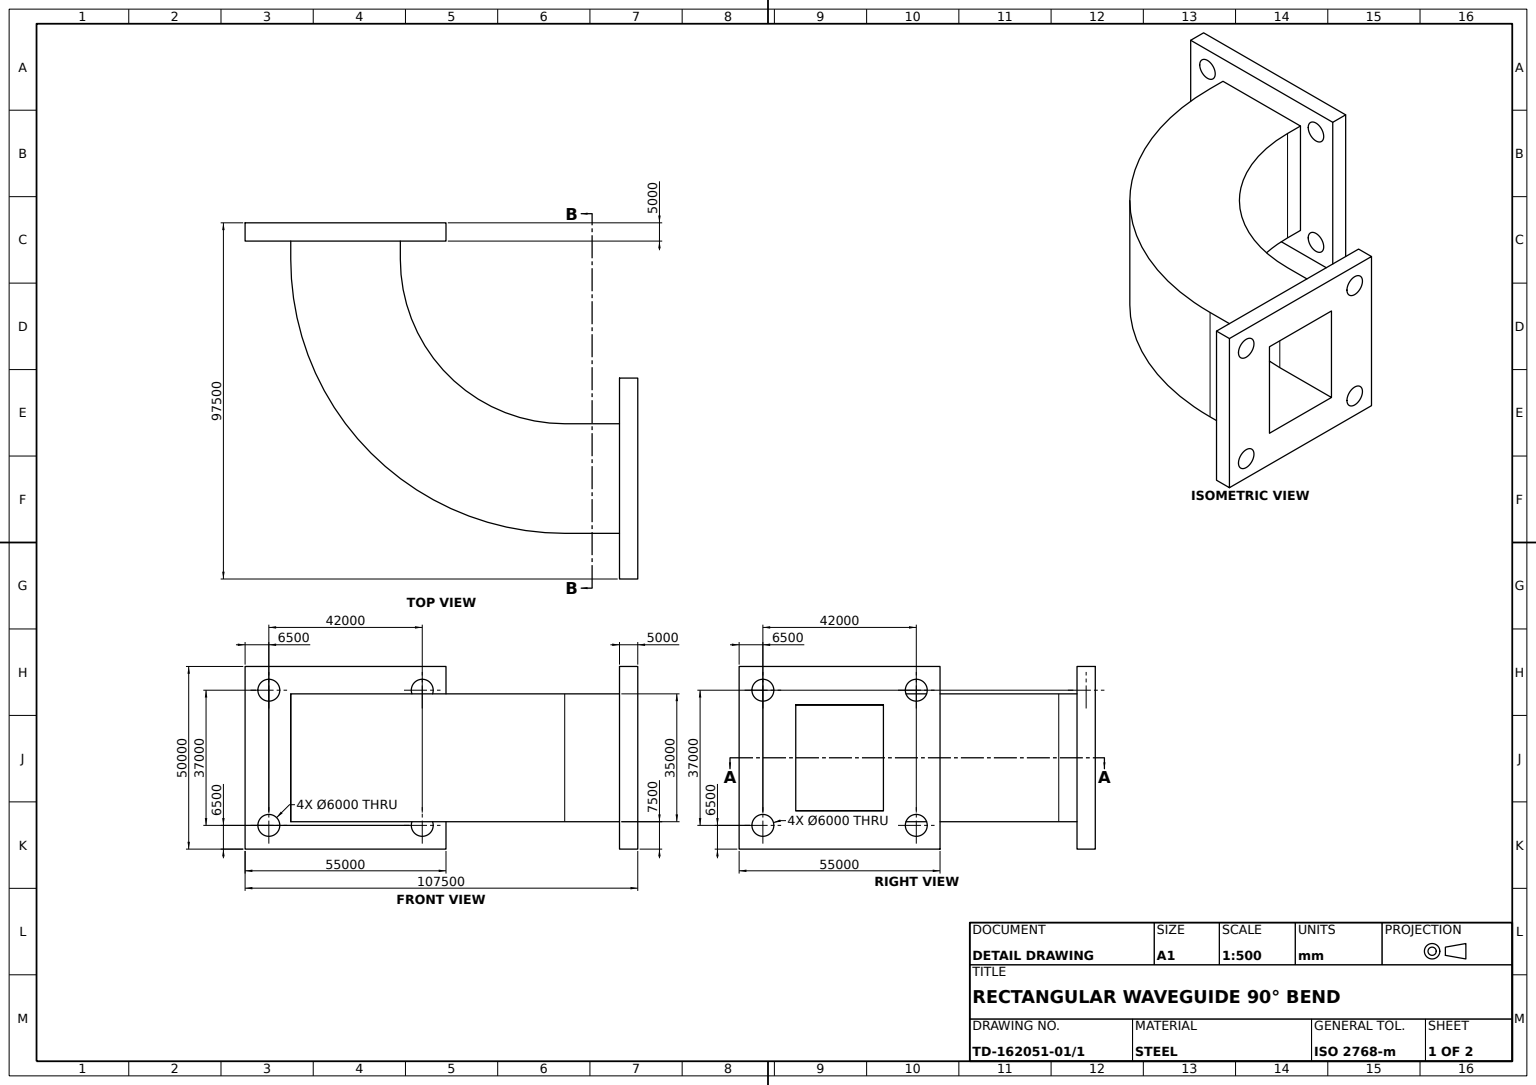
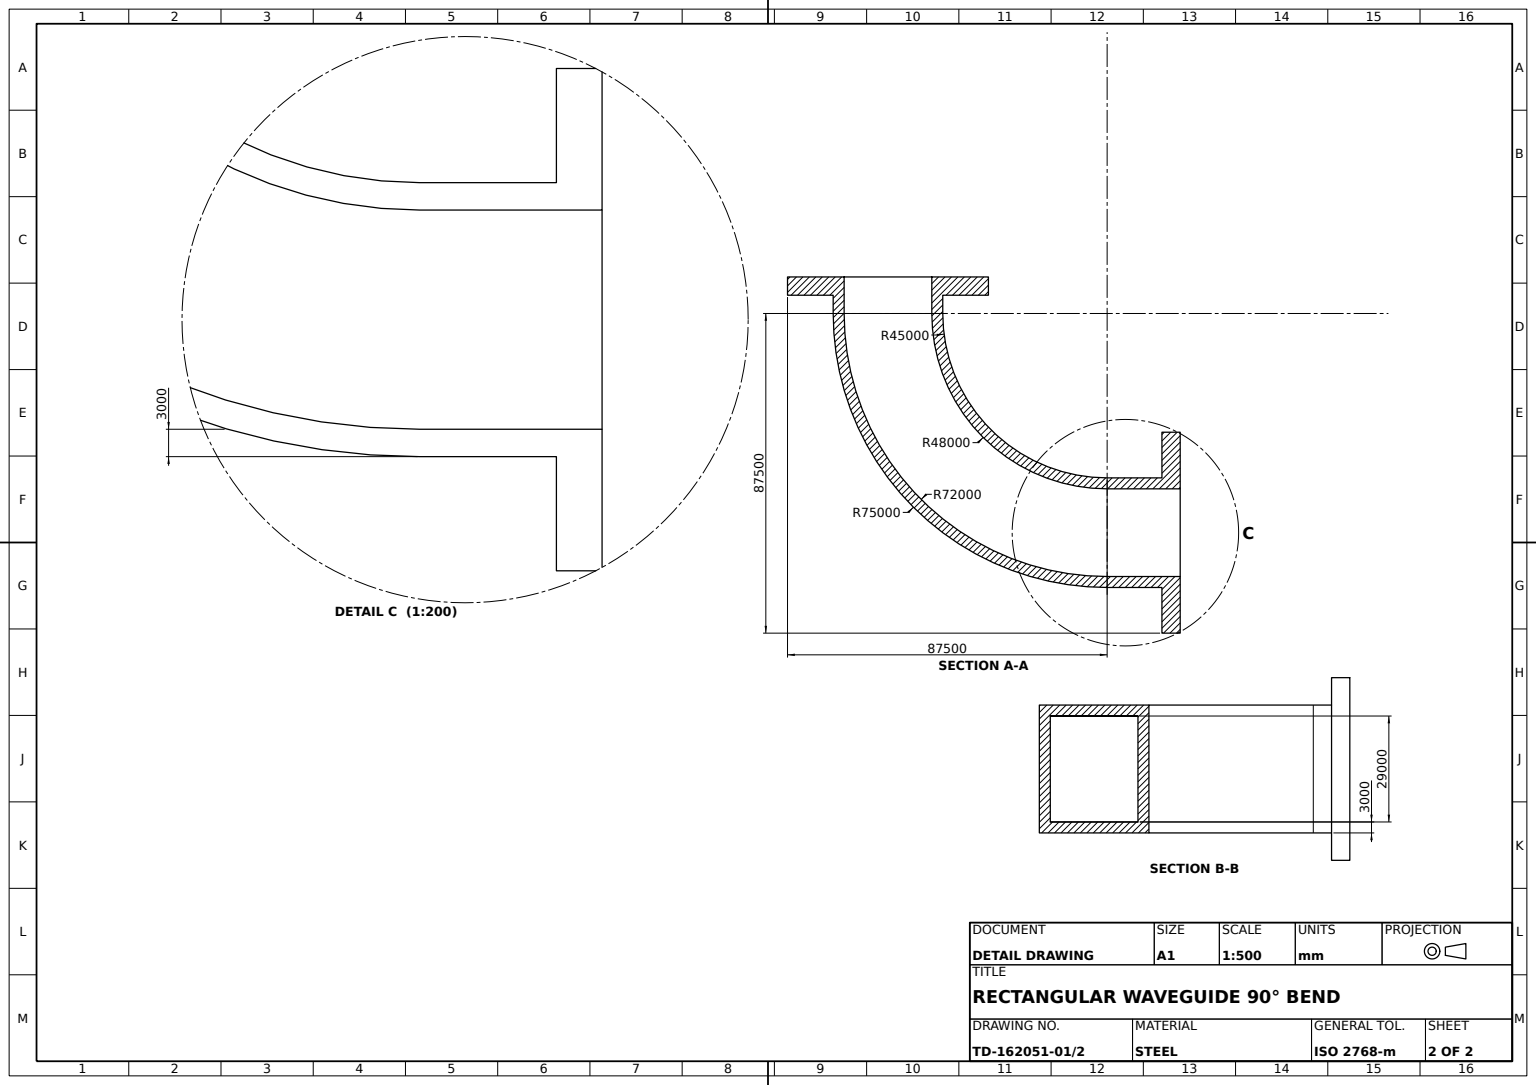
ISO-10303-21;
HEADER;
FILE_DESCRIPTION((''),'2;1');
FILE_NAME('','',(''),(''),'','','');
FILE_SCHEMA(('AUTOMOTIVE_DESIGN'));
ENDSEC;
DATA;
#1=APPLICATION_CONTEXT('');
#2=PRODUCT_CONTEXT('',#1,'mechanical');
#3=PRODUCT('','','',(#2));
#4=PRODUCT_DEFINITION_FORMATION('','',#3);
#5=PRODUCT_DEFINITION_CONTEXT('',#1,'design');
#6=PRODUCT_DEFINITION('','',#4,#5);
#7=PRODUCT_DEFINITION_SHAPE('','',#6);
#8=(LENGTH_UNIT()NAMED_UNIT(*)SI_UNIT(.MILLI.,.METRE.));
#9=(NAMED_UNIT(*)PLANE_ANGLE_UNIT()SI_UNIT($,.RADIAN.));
#10=(NAMED_UNIT(*)SI_UNIT($,.STERADIAN.)SOLID_ANGLE_UNIT());
#11=UNCERTAINTY_MEASURE_WITH_UNIT(LENGTH_MEASURE(1.E-05),#8,'distance_accuracy_value','');
#12=(GEOMETRIC_REPRESENTATION_CONTEXT(3)GLOBAL_UNCERTAINTY_ASSIGNED_CONTEXT((#11))GLOBAL_UNIT_ASSIGNED_CONTEXT((#8,#9,#10))REPRESENTATION_CONTEXT('',''));
#13=CARTESIAN_POINT('',(89000.,-18500.,-80000.));
#14=VERTEX_POINT('',#13);
#15=CARTESIAN_POINT('',(83000.,-18500.,-80000.));
#16=VERTEX_POINT('',#15);
#17=CARTESIAN_POINT('',(86000.,-18500.,-80000.));
#18=DIRECTION('',(0.,0.,-1.));
#19=DIRECTION('',(-1.,0.,0.));
#20=AXIS2_PLACEMENT_3D('',#17,#18,#19);
#21=CIRCLE('',#20,3000.);
#22=EDGE_CURVE('',#14,#16,#21,.T.);
#23=ORIENTED_EDGE('',*,*,#22,.T.);
#24=CARTESIAN_POINT('',(83000.,-18500.,-75000.));
#25=VERTEX_POINT('',#24);
#26=CARTESIAN_POINT('',(83000.,-18500.,27500.001));
#27=VECTOR('',#18,1000.);
#28=LINE('',#26,#27);
#29=EDGE_CURVE('',#25,#16,#28,.T.);
#30=ORIENTED_EDGE('',*,*,#29,.F.);
#31=CARTESIAN_POINT('',(89000.,-18500.,-75000.));
#32=VERTEX_POINT('',#31);
#33=CARTESIAN_POINT('',(86000.,-18500.,-75000.));
#34=DIRECTION('',(0.,0.,1.));
#35=AXIS2_PLACEMENT_3D('',#33,#34,#19);
#36=CIRCLE('',#35,3000.);
#37=EDGE_CURVE('',#25,#32,#36,.T.);
#38=ORIENTED_EDGE('',*,*,#37,.T.);
#39=CARTESIAN_POINT('',(89000.,-18500.,27500.001));
#40=LINE('',#39,#27);
#41=EDGE_CURVE('',#32,#14,#40,.T.);
#42=ORIENTED_EDGE('',*,*,#41,.T.);
#43=EDGE_LOOP('',(#23,#30,#38,#42));
#44=FACE_OUTER_BOUND('',#43,.T.);
#45=CARTESIAN_POINT('',(86000.,-18500.,27500.001));
#46=AXIS2_PLACEMENT_3D('',#45,#18,#19);
#47=CYLINDRICAL_SURFACE('',#46,3000.);
#48=ADVANCED_FACE('',(#44),#47,.F.);
#49=CARTESIAN_POINT('',(50000.,-17500.,-60000.));
#50=VERTEX_POINT('',#49);
#51=CARTESIAN_POINT('',(50000.,-17500.,-75000.));
#52=VERTEX_POINT('',#51);
#53=LINE('',#49,#27);
#54=EDGE_CURVE('',#50,#52,#53,.T.);
#55=ORIENTED_EDGE('',*,*,#54,.F.);
#56=CARTESIAN_POINT('',(50000.,17500.,-60000.));
#57=VERTEX_POINT('',#56);
#58=CARTESIAN_POINT('',(50000.,14500.,-60000.));
#59=DIRECTION('',(0.,1.,0.));
#60=VECTOR('',#59,1000.);
#61=LINE('',#58,#60);
#62=EDGE_CURVE('',#50,#57,#61,.T.);
#63=ORIENTED_EDGE('',*,*,#62,.T.);
#64=CARTESIAN_POINT('',(50000.,17500.,-75000.));
#65=VERTEX_POINT('',#64);
#66=LINE('',#56,#27);
#67=EDGE_CURVE('',#57,#65,#66,.T.);
#68=ORIENTED_EDGE('',*,*,#67,.T.);
#69=CARTESIAN_POINT('',(50000.,0.,-75000.));
#70=LINE('',#69,#60);
#71=EDGE_CURVE('',#52,#65,#70,.T.);
#72=ORIENTED_EDGE('',*,*,#71,.F.);
#73=EDGE_LOOP('',(#55,#63,#68,#72));
#74=FACE_OUTER_BOUND('',#73,.T.);
#75=DIRECTION('',(0.,-1.,0.));
#76=AXIS2_PLACEMENT_3D('',#58,#19,#75);
#77=PLANE('',#76);
#78=ADVANCED_FACE('',(#74),#77,.T.);
#79=CARTESIAN_POINT('',(80000.,-17500.,-60000.));
#80=VERTEX_POINT('',#79);
#81=CARTESIAN_POINT('',(77000.,-17500.,-60000.));
#82=VECTOR('',#19,1000.);
#83=LINE('',#81,#82);
#84=EDGE_CURVE('',#80,#50,#83,.T.);
#85=ORIENTED_EDGE('',*,*,#84,.F.);
#86=CARTESIAN_POINT('',(5000.,-17500.,15000.));
#87=VERTEX_POINT('',#86);
#88=CARTESIAN_POINT('',(5000.,-17500.,-60000.));
#89=AXIS2_PLACEMENT_3D('',#88,#59,#18);
#90=CIRCLE('',#89,75000.);
#91=EDGE_CURVE('',#87,#80,#90,.T.);
#92=ORIENTED_EDGE('',*,*,#91,.F.);
#93=CARTESIAN_POINT('',(5000.,-17500.,-15000.));
#94=VERTEX_POINT('',#93);
#95=CARTESIAN_POINT('',(5000.,-17500.,12000.));
#96=LINE('',#95,#27);
#97=EDGE_CURVE('',#87,#94,#96,.T.);
#98=ORIENTED_EDGE('',*,*,#97,.T.);
#99=CIRCLE('',#89,45000.);
#100=EDGE_CURVE('',#94,#50,#99,.T.);
#101=ORIENTED_EDGE('',*,*,#100,.T.);
#102=EDGE_LOOP('',(#85,#92,#98,#101));
#103=FACE_OUTER_BOUND('',#102,.T.);
#104=AXIS2_PLACEMENT_3D('',#95,#75,#18);
#105=PLANE('',#104);
#106=ADVANCED_FACE('',(#103),#105,.T.);
#107=CARTESIAN_POINT('',(0.,-18500.,-24000.));
#108=VERTEX_POINT('',#107);
#109=CARTESIAN_POINT('',(0.,-18500.,-18000.));
#110=VERTEX_POINT('',#109);
#111=CARTESIAN_POINT('',(0.,-18500.,-21000.));
#112=DIRECTION('',(1.,0.,0.));
#113=AXIS2_PLACEMENT_3D('',#111,#112,#34);
#114=CIRCLE('',#113,3000.);
#115=EDGE_CURVE('',#108,#110,#114,.T.);
#116=ORIENTED_EDGE('',*,*,#115,.T.);
#117=CARTESIAN_POINT('',(-5000.,-18500.,-18000.));
#118=VERTEX_POINT('',#117);
#119=CARTESIAN_POINT('',(92500.001,-18500.,-18000.));
#120=LINE('',#119,#82);
#121=EDGE_CURVE('',#110,#118,#120,.T.);
#122=ORIENTED_EDGE('',*,*,#121,.T.);
#123=CARTESIAN_POINT('',(-5000.,-18500.,-24000.));
#124=VERTEX_POINT('',#123);
#125=CARTESIAN_POINT('',(-5000.,-18500.,-21000.));
#126=AXIS2_PLACEMENT_3D('',#125,#19,#34);
#127=CIRCLE('',#126,3000.);
#128=EDGE_CURVE('',#118,#124,#127,.T.);
#129=ORIENTED_EDGE('',*,*,#128,.T.);
#130=CARTESIAN_POINT('',(92500.001,-18500.,-24000.));
#131=LINE('',#130,#82);
#132=EDGE_CURVE('',#108,#124,#131,.T.);
#133=ORIENTED_EDGE('',*,*,#132,.F.);
#134=EDGE_LOOP('',(#116,#122,#129,#133));
#135=FACE_OUTER_BOUND('',#134,.T.);
#136=CARTESIAN_POINT('',(92500.001,-18500.,-21000.));
#137=AXIS2_PLACEMENT_3D('',#136,#19,#34);
#138=CYLINDRICAL_SURFACE('',#137,3000.);
#139=ADVANCED_FACE('',(#135),#138,.F.);
#140=CARTESIAN_POINT('',(0.,17500.,15000.));
#141=VERTEX_POINT('',#140);
#142=CARTESIAN_POINT('',(0.,-17500.,15000.));
#143=VERTEX_POINT('',#142);
#144=CARTESIAN_POINT('',(0.,0.,15000.));
#145=VECTOR('',#75,1000.);
#146=LINE('',#144,#145);
#147=EDGE_CURVE('',#141,#143,#146,.T.);
#148=ORIENTED_EDGE('',*,*,#147,.F.);
#149=CARTESIAN_POINT('',(0.,17500.,-15000.));
#150=VERTEX_POINT('',#149);
#151=CARTESIAN_POINT('',(0.,17500.,0.));
#152=VECTOR('',#34,1000.);
#153=LINE('',#151,#152);
#154=EDGE_CURVE('',#150,#141,#153,.T.);
#155=ORIENTED_EDGE('',*,*,#154,.F.);
#156=CARTESIAN_POINT('',(0.,-17500.,-15000.));
#157=VERTEX_POINT('',#156);
#158=CARTESIAN_POINT('',(0.,0.,-15000.));
#159=LINE('',#158,#60);
#160=EDGE_CURVE('',#157,#150,#159,.T.);
#161=ORIENTED_EDGE('',*,*,#160,.F.);
#162=CARTESIAN_POINT('',(0.,-17500.,0.));
#163=LINE('',#162,#27);
#164=EDGE_CURVE('',#143,#157,#163,.T.);
#165=ORIENTED_EDGE('',*,*,#164,.F.);
#166=EDGE_LOOP('',(#148,#155,#161,#165));
#167=FACE_BOUND('',#166,.T.);
#168=CARTESIAN_POINT('',(0.,-25000.,-27500.));
#169=VERTEX_POINT('',#168);
#170=CARTESIAN_POINT('',(0.,-25000.,27500.));
#171=VERTEX_POINT('',#170);
#172=LINE('',#168,#152);
#173=EDGE_CURVE('',#169,#171,#172,.T.);
#174=ORIENTED_EDGE('',*,*,#173,.F.);
#175=CARTESIAN_POINT('',(0.,25000.,-27500.));
#176=VERTEX_POINT('',#175);
#177=LINE('',#175,#145);
#178=EDGE_CURVE('',#176,#169,#177,.T.);
#179=ORIENTED_EDGE('',*,*,#178,.F.);
#180=CARTESIAN_POINT('',(0.,25000.,27500.));
#181=VERTEX_POINT('',#180);
#182=LINE('',#175,#27);
#183=EDGE_CURVE('',#181,#176,#182,.T.);
#184=ORIENTED_EDGE('',*,*,#183,.F.);
#185=LINE('',#180,#60);
#186=EDGE_CURVE('',#171,#181,#185,.T.);
#187=ORIENTED_EDGE('',*,*,#186,.F.);
#188=EDGE_LOOP('',(#174,#179,#184,#187));
#189=FACE_OUTER_BOUND('',#188,.T.);
#190=ORIENTED_EDGE('',*,*,#115,.F.);
#191=EDGE_CURVE('',#110,#108,#114,.T.);
#192=ORIENTED_EDGE('',*,*,#191,.F.);
#193=EDGE_LOOP('',(#190,#192));
#194=FACE_BOUND('',#193,.T.);
#195=CARTESIAN_POINT('',(0.,18500.,18000.));
#196=VERTEX_POINT('',#195);
#197=CARTESIAN_POINT('',(0.,18500.,24000.));
#198=VERTEX_POINT('',#197);
#199=CARTESIAN_POINT('',(0.,18500.,21000.));
#200=AXIS2_PLACEMENT_3D('',#199,#112,#34);
#201=CIRCLE('',#200,3000.);
#202=EDGE_CURVE('',#196,#198,#201,.T.);
#203=ORIENTED_EDGE('',*,*,#202,.F.);
#204=EDGE_CURVE('',#198,#196,#201,.T.);
#205=ORIENTED_EDGE('',*,*,#204,.F.);
#206=EDGE_LOOP('',(#203,#205));
#207=FACE_BOUND('',#206,.T.);
#208=CARTESIAN_POINT('',(0.,18500.,-24000.));
#209=VERTEX_POINT('',#208);
#210=CARTESIAN_POINT('',(0.,18500.,-18000.));
#211=VERTEX_POINT('',#210);
#212=CARTESIAN_POINT('',(0.,18500.,-21000.));
#213=AXIS2_PLACEMENT_3D('',#212,#112,#34);
#214=CIRCLE('',#213,3000.);
#215=EDGE_CURVE('',#209,#211,#214,.T.);
#216=ORIENTED_EDGE('',*,*,#215,.F.);
#217=EDGE_CURVE('',#211,#209,#214,.T.);
#218=ORIENTED_EDGE('',*,*,#217,.F.);
#219=EDGE_LOOP('',(#216,#218));
#220=FACE_BOUND('',#219,.T.);
#221=CARTESIAN_POINT('',(0.,-18500.,24000.));
#222=VERTEX_POINT('',#221);
#223=CARTESIAN_POINT('',(0.,-18500.,18000.));
#224=VERTEX_POINT('',#223);
#225=CARTESIAN_POINT('',(0.,-18500.,21000.));
#226=AXIS2_PLACEMENT_3D('',#225,#112,#34);
#227=CIRCLE('',#226,3000.);
#228=EDGE_CURVE('',#222,#224,#227,.T.);
#229=ORIENTED_EDGE('',*,*,#228,.F.);
#230=EDGE_CURVE('',#224,#222,#227,.T.);
#231=ORIENTED_EDGE('',*,*,#230,.F.);
#232=EDGE_LOOP('',(#229,#231));
#233=FACE_BOUND('',#232,.T.);
#234=CARTESIAN_POINT('',(0.,0.,0.));
#235=AXIS2_PLACEMENT_3D('',#234,#19,#34);
#236=PLANE('',#235);
#237=ADVANCED_FACE('',(#167,#189,#194,#207,#220,#233),#236,.F.);
#238=CARTESIAN_POINT('',(80000.,17500.,-60000.));
#239=VERTEX_POINT('',#238);
#240=CARTESIAN_POINT('',(80000.,17500.,-75000.));
#241=VERTEX_POINT('',#240);
#242=LINE('',#238,#27);
#243=EDGE_CURVE('',#239,#241,#242,.T.);
#244=ORIENTED_EDGE('',*,*,#243,.F.);
#245=CARTESIAN_POINT('',(80000.,14500.,-60000.));
#246=LINE('',#245,#145);
#247=EDGE_CURVE('',#239,#80,#246,.T.);
#248=ORIENTED_EDGE('',*,*,#247,.T.);
#249=CARTESIAN_POINT('',(80000.,-17500.,-75000.));
#250=VERTEX_POINT('',#249);
#251=LINE('',#79,#27);
#252=EDGE_CURVE('',#80,#250,#251,.T.);
#253=ORIENTED_EDGE('',*,*,#252,.T.);
#254=CARTESIAN_POINT('',(80000.,0.,-75000.));
#255=LINE('',#254,#145);
#256=EDGE_CURVE('',#241,#250,#255,.T.);
#257=ORIENTED_EDGE('',*,*,#256,.F.);
#258=EDGE_LOOP('',(#244,#248,#253,#257));
#259=FACE_OUTER_BOUND('',#258,.T.);
#260=AXIS2_PLACEMENT_3D('',#245,#112,#59);
#261=PLANE('',#260);
#262=ADVANCED_FACE('',(#259),#261,.T.);
#263=CARTESIAN_POINT('',(5000.,17500.,-15000.));
#264=VERTEX_POINT('',#263);
#265=CARTESIAN_POINT('',(5000.,17500.,-60000.));
#266=AXIS2_PLACEMENT_3D('',#265,#59,#34);
#267=CIRCLE('',#266,45000.);
#268=EDGE_CURVE('',#264,#57,#267,.T.);
#269=ORIENTED_EDGE('',*,*,#268,.F.);
#270=CARTESIAN_POINT('',(5000.,17500.,15000.));
#271=VERTEX_POINT('',#270);
#272=CARTESIAN_POINT('',(5000.,17500.,12000.));
#273=LINE('',#272,#152);
#274=EDGE_CURVE('',#264,#271,#273,.T.);
#275=ORIENTED_EDGE('',*,*,#274,.T.);
#276=CIRCLE('',#266,75000.);
#277=EDGE_CURVE('',#271,#239,#276,.T.);
#278=ORIENTED_EDGE('',*,*,#277,.T.);
#279=CARTESIAN_POINT('',(77000.,17500.,-60000.));
#280=VECTOR('',#112,1000.);
#281=LINE('',#279,#280);
#282=EDGE_CURVE('',#57,#239,#281,.T.);
#283=ORIENTED_EDGE('',*,*,#282,.F.);
#284=EDGE_LOOP('',(#269,#275,#278,#283));
#285=FACE_OUTER_BOUND('',#284,.T.);
#286=AXIS2_PLACEMENT_3D('',#272,#59,#34);
#287=PLANE('',#286);
#288=ADVANCED_FACE('',(#285),#287,.T.);
#289=ORIENTED_EDGE('',*,*,#217,.T.);
#290=CARTESIAN_POINT('',(-5000.,18500.,-24000.));
#291=VERTEX_POINT('',#290);
#292=CARTESIAN_POINT('',(92500.001,18500.,-24000.));
#293=LINE('',#292,#82);
#294=EDGE_CURVE('',#209,#291,#293,.T.);
#295=ORIENTED_EDGE('',*,*,#294,.T.);
#296=CARTESIAN_POINT('',(-5000.,18500.,-18000.));
#297=VERTEX_POINT('',#296);
#298=CARTESIAN_POINT('',(-5000.,18500.,-21000.));
#299=AXIS2_PLACEMENT_3D('',#298,#19,#34);
#300=CIRCLE('',#299,3000.);
#301=EDGE_CURVE('',#291,#297,#300,.T.);
#302=ORIENTED_EDGE('',*,*,#301,.T.);
#303=CARTESIAN_POINT('',(92500.001,18500.,-18000.));
#304=LINE('',#303,#82);
#305=EDGE_CURVE('',#211,#297,#304,.T.);
#306=ORIENTED_EDGE('',*,*,#305,.F.);
#307=EDGE_LOOP('',(#289,#295,#302,#306));
#308=FACE_OUTER_BOUND('',#307,.T.);
#309=CARTESIAN_POINT('',(92500.001,18500.,-21000.));
#310=AXIS2_PLACEMENT_3D('',#309,#19,#34);
#311=CYLINDRICAL_SURFACE('',#310,3000.);
#312=ADVANCED_FACE('',(#308),#311,.F.);
#313=CARTESIAN_POINT('',(41000.,18500.,-75000.));
#314=VERTEX_POINT('',#313);
#315=CARTESIAN_POINT('',(41000.,18500.,-80000.));
#316=VERTEX_POINT('',#315);
#317=CARTESIAN_POINT('',(41000.,18500.,27500.001));
#318=LINE('',#317,#27);
#319=EDGE_CURVE('',#314,#316,#318,.T.);
#320=ORIENTED_EDGE('',*,*,#319,.T.);
#321=CARTESIAN_POINT('',(47000.,18500.,-80000.));
#322=VERTEX_POINT('',#321);
#323=CARTESIAN_POINT('',(44000.,18500.,-80000.));
#324=AXIS2_PLACEMENT_3D('',#323,#18,#19);
#325=CIRCLE('',#324,3000.);
#326=EDGE_CURVE('',#316,#322,#325,.T.);
#327=ORIENTED_EDGE('',*,*,#326,.T.);
#328=CARTESIAN_POINT('',(47000.,18500.,-75000.));
#329=VERTEX_POINT('',#328);
#330=CARTESIAN_POINT('',(47000.,18500.,27500.001));
#331=LINE('',#330,#27);
#332=EDGE_CURVE('',#329,#322,#331,.T.);
#333=ORIENTED_EDGE('',*,*,#332,.F.);
#334=CARTESIAN_POINT('',(44000.,18500.,-75000.));
#335=AXIS2_PLACEMENT_3D('',#334,#34,#19);
#336=CIRCLE('',#335,3000.);
#337=EDGE_CURVE('',#329,#314,#336,.T.);
#338=ORIENTED_EDGE('',*,*,#337,.T.);
#339=EDGE_LOOP('',(#320,#327,#333,#338));
#340=FACE_OUTER_BOUND('',#339,.T.);
#341=CARTESIAN_POINT('',(44000.,18500.,27500.001));
#342=AXIS2_PLACEMENT_3D('',#341,#18,#19);
#343=CYLINDRICAL_SURFACE('',#342,3000.);
#344=ADVANCED_FACE('',(#340),#343,.F.);
#345=CARTESIAN_POINT('',(5000.,0.,-15000.));
#346=LINE('',#345,#60);
#347=EDGE_CURVE('',#94,#264,#346,.T.);
#348=ORIENTED_EDGE('',*,*,#347,.T.);
#349=ORIENTED_EDGE('',*,*,#268,.T.);
#350=ORIENTED_EDGE('',*,*,#62,.F.);
#351=ORIENTED_EDGE('',*,*,#100,.F.);
#352=EDGE_LOOP('',(#348,#349,#350,#351));
#353=FACE_OUTER_BOUND('',#352,.T.);
#354=CARTESIAN_POINT('',(5000.,0.,-60000.));
#355=AXIS2_PLACEMENT_3D('',#354,#59,#34);
#356=CYLINDRICAL_SURFACE('',#355,45000.);
#357=ADVANCED_FACE('',(#353),#356,.F.);
#358=CARTESIAN_POINT('',(83000.,18500.,-75000.));
#359=VERTEX_POINT('',#358);
#360=CARTESIAN_POINT('',(83000.,18500.,-80000.));
#361=VERTEX_POINT('',#360);
#362=CARTESIAN_POINT('',(83000.,18500.,27500.001));
#363=LINE('',#362,#27);
#364=EDGE_CURVE('',#359,#361,#363,.T.);
#365=ORIENTED_EDGE('',*,*,#364,.T.);
#366=CARTESIAN_POINT('',(89000.,18500.,-80000.));
#367=VERTEX_POINT('',#366);
#368=CARTESIAN_POINT('',(86000.,18500.,-80000.));
#369=AXIS2_PLACEMENT_3D('',#368,#18,#19);
#370=CIRCLE('',#369,3000.);
#371=EDGE_CURVE('',#361,#367,#370,.T.);
#372=ORIENTED_EDGE('',*,*,#371,.T.);
#373=CARTESIAN_POINT('',(89000.,18500.,-75000.));
#374=VERTEX_POINT('',#373);
#375=CARTESIAN_POINT('',(89000.,18500.,27500.001));
#376=LINE('',#375,#27);
#377=EDGE_CURVE('',#374,#367,#376,.T.);
#378=ORIENTED_EDGE('',*,*,#377,.F.);
#379=CARTESIAN_POINT('',(86000.,18500.,-75000.));
#380=AXIS2_PLACEMENT_3D('',#379,#34,#19);
#381=CIRCLE('',#380,3000.);
#382=EDGE_CURVE('',#374,#359,#381,.T.);
#383=ORIENTED_EDGE('',*,*,#382,.T.);
#384=EDGE_LOOP('',(#365,#372,#378,#383));
#385=FACE_OUTER_BOUND('',#384,.T.);
#386=CARTESIAN_POINT('',(86000.,18500.,27500.001));
#387=AXIS2_PLACEMENT_3D('',#386,#18,#19);
#388=CYLINDRICAL_SURFACE('',#387,3000.);
#389=ADVANCED_FACE('',(#385),#388,.F.);
#390=LINE('',#140,#280);
#391=EDGE_CURVE('',#141,#271,#390,.T.);
#392=ORIENTED_EDGE('',*,*,#391,.T.);
#393=ORIENTED_EDGE('',*,*,#274,.F.);
#394=LINE('',#149,#280);
#395=EDGE_CURVE('',#150,#264,#394,.T.);
#396=ORIENTED_EDGE('',*,*,#395,.F.);
#397=ORIENTED_EDGE('',*,*,#154,.T.);
#398=EDGE_LOOP('',(#392,#393,#396,#397));
#399=FACE_OUTER_BOUND('',#398,.T.);
#400=CARTESIAN_POINT('',(0.,17500.,12000.));
#401=AXIS2_PLACEMENT_3D('',#400,#59,#34);
#402=PLANE('',#401);
#403=ADVANCED_FACE('',(#399),#402,.T.);
#404=CARTESIAN_POINT('',(-5000.,-14500.,12000.));
#405=VERTEX_POINT('',#404);
#406=CARTESIAN_POINT('',(5000.,-14500.,12000.));
#407=VERTEX_POINT('',#406);
#408=CARTESIAN_POINT('',(0.,-14500.,12000.));
#409=LINE('',#408,#280);
#410=EDGE_CURVE('',#405,#407,#409,.T.);
#411=ORIENTED_EDGE('',*,*,#410,.F.);
#412=CARTESIAN_POINT('',(-5000.,14500.,12000.));
#413=VERTEX_POINT('',#412);
#414=LINE('',#412,#60);
#415=EDGE_CURVE('',#405,#413,#414,.T.);
#416=ORIENTED_EDGE('',*,*,#415,.T.);
#417=CARTESIAN_POINT('',(5000.,14500.,12000.));
#418=VERTEX_POINT('',#417);
#419=CARTESIAN_POINT('',(0.,14500.,12000.));
#420=LINE('',#419,#280);
#421=EDGE_CURVE('',#413,#418,#420,.T.);
#422=ORIENTED_EDGE('',*,*,#421,.T.);
#423=LINE('',#417,#145);
#424=EDGE_CURVE('',#418,#407,#423,.T.);
#425=ORIENTED_EDGE('',*,*,#424,.T.);
#426=EDGE_LOOP('',(#411,#416,#422,#425));
#427=FACE_OUTER_BOUND('',#426,.T.);
#428=AXIS2_PLACEMENT_3D('',#419,#34,#75);
#429=PLANE('',#428);
#430=ADVANCED_FACE('',(#427),#429,.F.);
#431=CARTESIAN_POINT('',(-5000.,25000.,27500.));
#432=VERTEX_POINT('',#431);
#433=LINE('',#431,#280);
#434=EDGE_CURVE('',#432,#181,#433,.T.);
#435=ORIENTED_EDGE('',*,*,#434,.F.);
#436=CARTESIAN_POINT('',(-5000.,-25000.,27500.));
#437=VERTEX_POINT('',#436);
#438=LINE('',#431,#60);
#439=EDGE_CURVE('',#437,#432,#438,.T.);
#440=ORIENTED_EDGE('',*,*,#439,.F.);
#441=LINE('',#436,#280);
#442=EDGE_CURVE('',#437,#171,#441,.T.);
#443=ORIENTED_EDGE('',*,*,#442,.T.);
#444=ORIENTED_EDGE('',*,*,#186,.T.);
#445=EDGE_LOOP('',(#435,#440,#443,#444));
#446=FACE_OUTER_BOUND('',#445,.T.);
#447=AXIS2_PLACEMENT_3D('',#431,#18,#59);
#448=PLANE('',#447);
#449=ADVANCED_FACE('',(#446),#448,.F.);
#450=CARTESIAN_POINT('',(77000.,-14500.,-60000.));
#451=VERTEX_POINT('',#450);
#452=CARTESIAN_POINT('',(77000.,-14500.,-80000.));
#453=VERTEX_POINT('',#452);
#454=LINE('',#450,#27);
#455=EDGE_CURVE('',#451,#453,#454,.T.);
#456=ORIENTED_EDGE('',*,*,#455,.T.);
#457=CARTESIAN_POINT('',(53000.,-14500.,-80000.));
#458=VERTEX_POINT('',#457);
#459=LINE('',#452,#82);
#460=EDGE_CURVE('',#453,#458,#459,.T.);
#461=ORIENTED_EDGE('',*,*,#460,.T.);
#462=CARTESIAN_POINT('',(53000.,-14500.,-60000.));
#463=VERTEX_POINT('',#462);
#464=LINE('',#462,#27);
#465=EDGE_CURVE('',#463,#458,#464,.T.);
#466=ORIENTED_EDGE('',*,*,#465,.F.);
#467=LINE('',#450,#82);
#468=EDGE_CURVE('',#451,#463,#467,.T.);
#469=ORIENTED_EDGE('',*,*,#468,.F.);
#470=EDGE_LOOP('',(#456,#461,#466,#469));
#471=FACE_OUTER_BOUND('',#470,.T.);
#472=AXIS2_PLACEMENT_3D('',#450,#75,#18);
#473=PLANE('',#472);
#474=ADVANCED_FACE('',(#471),#473,.F.);
#475=CARTESIAN_POINT('',(37500.,25000.,-80000.));
#476=VERTEX_POINT('',#475);
#477=CARTESIAN_POINT('',(92500.,25000.,-80000.));
#478=VERTEX_POINT('',#477);
#479=LINE('',#477,#280);
#480=EDGE_CURVE('',#476,#478,#479,.T.);
#481=ORIENTED_EDGE('',*,*,#480,.F.);
#482=CARTESIAN_POINT('',(37500.,25000.,-75000.));
#483=VERTEX_POINT('',#482);
#484=LINE('',#475,#152);
#485=EDGE_CURVE('',#476,#483,#484,.T.);
#486=ORIENTED_EDGE('',*,*,#485,.T.);
#487=CARTESIAN_POINT('',(92500.,25000.,-75000.));
#488=VERTEX_POINT('',#487);
#489=LINE('',#487,#280);
#490=EDGE_CURVE('',#483,#488,#489,.T.);
#491=ORIENTED_EDGE('',*,*,#490,.T.);
#492=LINE('',#477,#152);
#493=EDGE_CURVE('',#478,#488,#492,.T.);
#494=ORIENTED_EDGE('',*,*,#493,.F.);
#495=EDGE_LOOP('',(#481,#486,#491,#494));
#496=FACE_OUTER_BOUND('',#495,.T.);
#497=AXIS2_PLACEMENT_3D('',#477,#75,#18);
#498=PLANE('',#497);
#499=ADVANCED_FACE('',(#496),#498,.F.);
#500=ORIENTED_EDGE('',*,*,#395,.T.);
#501=ORIENTED_EDGE('',*,*,#347,.F.);
#502=LINE('',#156,#280);
#503=EDGE_CURVE('',#157,#94,#502,.T.);
#504=ORIENTED_EDGE('',*,*,#503,.F.);
#505=ORIENTED_EDGE('',*,*,#160,.T.);
#506=EDGE_LOOP('',(#500,#501,#504,#505));
#507=FACE_OUTER_BOUND('',#506,.T.);
#508=CARTESIAN_POINT('',(0.,14500.,-15000.));
#509=AXIS2_PLACEMENT_3D('',#508,#18,#59);
#510=PLANE('',#509);
#511=ADVANCED_FACE('',(#507),#510,.T.);
#512=CARTESIAN_POINT('',(-5000.,18500.,24000.));
#513=VERTEX_POINT('',#512);
#514=CARTESIAN_POINT('',(92500.001,18500.,24000.));
#515=LINE('',#514,#82);
#516=EDGE_CURVE('',#198,#513,#515,.T.);
#517=ORIENTED_EDGE('',*,*,#516,.F.);
#518=ORIENTED_EDGE('',*,*,#204,.T.);
#519=CARTESIAN_POINT('',(-5000.,18500.,18000.));
#520=VERTEX_POINT('',#519);
#521=CARTESIAN_POINT('',(92500.001,18500.,18000.));
#522=LINE('',#521,#82);
#523=EDGE_CURVE('',#196,#520,#522,.T.);
#524=ORIENTED_EDGE('',*,*,#523,.T.);
#525=CARTESIAN_POINT('',(-5000.,18500.,21000.));
#526=AXIS2_PLACEMENT_3D('',#525,#19,#34);
#527=CIRCLE('',#526,3000.);
#528=EDGE_CURVE('',#520,#513,#527,.T.);
#529=ORIENTED_EDGE('',*,*,#528,.T.);
#530=EDGE_LOOP('',(#517,#518,#524,#529));
#531=FACE_OUTER_BOUND('',#530,.T.);
#532=CARTESIAN_POINT('',(92500.001,18500.,21000.));
#533=AXIS2_PLACEMENT_3D('',#532,#19,#34);
#534=CYLINDRICAL_SURFACE('',#533,3000.);
#535=ADVANCED_FACE('',(#531),#534,.F.);
#536=ORIENTED_EDGE('',*,*,#173,.T.);
#537=ORIENTED_EDGE('',*,*,#442,.F.);
#538=CARTESIAN_POINT('',(-5000.,-25000.,-27500.));
#539=VERTEX_POINT('',#538);
#540=LINE('',#538,#152);
#541=EDGE_CURVE('',#539,#437,#540,.T.);
#542=ORIENTED_EDGE('',*,*,#541,.F.);
#543=LINE('',#538,#280);
#544=EDGE_CURVE('',#539,#169,#543,.T.);
#545=ORIENTED_EDGE('',*,*,#544,.T.);
#546=EDGE_LOOP('',(#536,#537,#542,#545));
#547=FACE_OUTER_BOUND('',#546,.T.);
#548=AXIS2_PLACEMENT_3D('',#538,#59,#34);
#549=PLANE('',#548);
#550=ADVANCED_FACE('',(#547),#549,.F.);
#551=ORIENTED_EDGE('',*,*,#97,.F.);
#552=LINE('',#142,#280);
#553=EDGE_CURVE('',#143,#87,#552,.T.);
#554=ORIENTED_EDGE('',*,*,#553,.F.);
#555=ORIENTED_EDGE('',*,*,#164,.T.);
#556=ORIENTED_EDGE('',*,*,#503,.T.);
#557=EDGE_LOOP('',(#551,#554,#555,#556));
#558=FACE_OUTER_BOUND('',#557,.T.);
#559=CARTESIAN_POINT('',(0.,-17500.,12000.));
#560=AXIS2_PLACEMENT_3D('',#559,#75,#18);
#561=PLANE('',#560);
#562=ADVANCED_FACE('',(#558),#561,.T.);
#563=CARTESIAN_POINT('',(41000.,-18500.,-75000.));
#564=VERTEX_POINT('',#563);
#565=CARTESIAN_POINT('',(41000.,-18500.,-80000.));
#566=VERTEX_POINT('',#565);
#567=CARTESIAN_POINT('',(41000.,-18500.,27500.001));
#568=LINE('',#567,#27);
#569=EDGE_CURVE('',#564,#566,#568,.T.);
#570=ORIENTED_EDGE('',*,*,#569,.F.);
#571=CARTESIAN_POINT('',(47000.,-18500.,-75000.));
#572=VERTEX_POINT('',#571);
#573=CARTESIAN_POINT('',(44000.,-18500.,-75000.));
#574=AXIS2_PLACEMENT_3D('',#573,#34,#19);
#575=CIRCLE('',#574,3000.);
#576=EDGE_CURVE('',#564,#572,#575,.T.);
#577=ORIENTED_EDGE('',*,*,#576,.T.);
#578=CARTESIAN_POINT('',(47000.,-18500.,-80000.));
#579=VERTEX_POINT('',#578);
#580=CARTESIAN_POINT('',(47000.,-18500.,27500.001));
#581=LINE('',#580,#27);
#582=EDGE_CURVE('',#572,#579,#581,.T.);
#583=ORIENTED_EDGE('',*,*,#582,.T.);
#584=CARTESIAN_POINT('',(44000.,-18500.,-80000.));
#585=AXIS2_PLACEMENT_3D('',#584,#18,#19);
#586=CIRCLE('',#585,3000.);
#587=EDGE_CURVE('',#579,#566,#586,.T.);
#588=ORIENTED_EDGE('',*,*,#587,.T.);
#589=EDGE_LOOP('',(#570,#577,#583,#588));
#590=FACE_OUTER_BOUND('',#589,.T.);
#591=CARTESIAN_POINT('',(44000.,-18500.,27500.001));
#592=AXIS2_PLACEMENT_3D('',#591,#18,#19);
#593=CYLINDRICAL_SURFACE('',#592,3000.);
#594=ADVANCED_FACE('',(#590),#593,.F.);
#595=CARTESIAN_POINT('',(77000.,14500.,-60000.));
#596=VERTEX_POINT('',#595);
#597=CARTESIAN_POINT('',(77000.,14500.,-80000.));
#598=VERTEX_POINT('',#597);
#599=LINE('',#595,#27);
#600=EDGE_CURVE('',#596,#598,#599,.T.);
#601=ORIENTED_EDGE('',*,*,#600,.T.);
#602=LINE('',#597,#145);
#603=EDGE_CURVE('',#598,#453,#602,.T.);
#604=ORIENTED_EDGE('',*,*,#603,.T.);
#605=ORIENTED_EDGE('',*,*,#455,.F.);
#606=LINE('',#595,#145);
#607=EDGE_CURVE('',#596,#451,#606,.T.);
#608=ORIENTED_EDGE('',*,*,#607,.F.);
#609=EDGE_LOOP('',(#601,#604,#605,#608));
#610=FACE_OUTER_BOUND('',#609,.T.);
#611=AXIS2_PLACEMENT_3D('',#595,#112,#59);
#612=PLANE('',#611);
#613=ADVANCED_FACE('',(#610),#612,.F.);
#614=CARTESIAN_POINT('',(-5000.,14500.,-12000.));
#615=VERTEX_POINT('',#614);
#616=LINE('',#614,#27);
#617=EDGE_CURVE('',#413,#615,#616,.T.);
#618=ORIENTED_EDGE('',*,*,#617,.T.);
#619=CARTESIAN_POINT('',(5000.,14500.,-12000.));
#620=VERTEX_POINT('',#619);
#621=CARTESIAN_POINT('',(0.,14500.,-12000.));
#622=LINE('',#621,#280);
#623=EDGE_CURVE('',#615,#620,#622,.T.);
#624=ORIENTED_EDGE('',*,*,#623,.T.);
#625=LINE('',#417,#152);
#626=EDGE_CURVE('',#620,#418,#625,.T.);
#627=ORIENTED_EDGE('',*,*,#626,.T.);
#628=ORIENTED_EDGE('',*,*,#421,.F.);
#629=EDGE_LOOP('',(#618,#624,#627,#628));
#630=FACE_OUTER_BOUND('',#629,.T.);
#631=AXIS2_PLACEMENT_3D('',#419,#59,#34);
#632=PLANE('',#631);
#633=ADVANCED_FACE('',(#630),#632,.F.);
#634=CARTESIAN_POINT('',(-5000.,-18500.,18000.));
#635=VERTEX_POINT('',#634);
#636=CARTESIAN_POINT('',(92500.001,-18500.,18000.));
#637=LINE('',#636,#82);
#638=EDGE_CURVE('',#224,#635,#637,.T.);
#639=ORIENTED_EDGE('',*,*,#638,.T.);
#640=CARTESIAN_POINT('',(-5000.,-18500.,24000.));
#641=VERTEX_POINT('',#640);
#642=CARTESIAN_POINT('',(-5000.,-18500.,21000.));
#643=AXIS2_PLACEMENT_3D('',#642,#19,#34);
#644=CIRCLE('',#643,3000.);
#645=EDGE_CURVE('',#635,#641,#644,.T.);
#646=ORIENTED_EDGE('',*,*,#645,.T.);
#647=CARTESIAN_POINT('',(92500.001,-18500.,24000.));
#648=LINE('',#647,#82);
#649=EDGE_CURVE('',#222,#641,#648,.T.);
#650=ORIENTED_EDGE('',*,*,#649,.F.);
#651=ORIENTED_EDGE('',*,*,#228,.T.);
#652=EDGE_LOOP('',(#639,#646,#650,#651));
#653=FACE_OUTER_BOUND('',#652,.T.);
#654=CARTESIAN_POINT('',(92500.001,-18500.,21000.));
#655=AXIS2_PLACEMENT_3D('',#654,#19,#34);
#656=CYLINDRICAL_SURFACE('',#655,3000.);
#657=ADVANCED_FACE('',(#653),#656,.F.);
#658=ORIENTED_EDGE('',*,*,#485,.F.);
#659=CARTESIAN_POINT('',(37500.,-25000.,-80000.));
#660=VERTEX_POINT('',#659);
#661=LINE('',#475,#60);
#662=EDGE_CURVE('',#660,#476,#661,.T.);
#663=ORIENTED_EDGE('',*,*,#662,.F.);
#664=CARTESIAN_POINT('',(37500.,-25000.,-75000.));
#665=VERTEX_POINT('',#664);
#666=LINE('',#659,#152);
#667=EDGE_CURVE('',#660,#665,#666,.T.);
#668=ORIENTED_EDGE('',*,*,#667,.T.);
#669=LINE('',#482,#60);
#670=EDGE_CURVE('',#665,#483,#669,.T.);
#671=ORIENTED_EDGE('',*,*,#670,.T.);
#672=EDGE_LOOP('',(#658,#663,#668,#671));
#673=FACE_OUTER_BOUND('',#672,.T.);
#674=AXIS2_PLACEMENT_3D('',#475,#112,#18);
#675=PLANE('',#674);
#676=ADVANCED_FACE('',(#673),#675,.F.);
#677=ORIENTED_EDGE('',*,*,#41,.F.);
#678=EDGE_CURVE('',#32,#25,#36,.T.);
#679=ORIENTED_EDGE('',*,*,#678,.T.);
#680=ORIENTED_EDGE('',*,*,#29,.T.);
#681=EDGE_CURVE('',#16,#14,#21,.T.);
#682=ORIENTED_EDGE('',*,*,#681,.T.);
#683=EDGE_LOOP('',(#677,#679,#680,#682));
#684=FACE_OUTER_BOUND('',#683,.T.);
#685=ADVANCED_FACE('',(#684),#47,.F.);
#686=ORIENTED_EDGE('',*,*,#382,.F.);
#687=EDGE_CURVE('',#359,#374,#381,.T.);
#688=ORIENTED_EDGE('',*,*,#687,.F.);
#689=EDGE_LOOP('',(#686,#688));
#690=FACE_BOUND('',#689,.T.);
#691=ORIENTED_EDGE('',*,*,#337,.F.);
#692=EDGE_CURVE('',#314,#329,#336,.T.);
#693=ORIENTED_EDGE('',*,*,#692,.F.);
#694=EDGE_LOOP('',(#691,#693));
#695=FACE_BOUND('',#694,.T.);
#696=EDGE_CURVE('',#572,#564,#575,.T.);
#697=ORIENTED_EDGE('',*,*,#696,.F.);
#698=ORIENTED_EDGE('',*,*,#576,.F.);
#699=EDGE_LOOP('',(#697,#698));
#700=FACE_BOUND('',#699,.T.);
#701=ORIENTED_EDGE('',*,*,#256,.T.);
#702=CARTESIAN_POINT('',(65000.,-17500.,-75000.));
#703=LINE('',#702,#82);
#704=EDGE_CURVE('',#250,#52,#703,.T.);
#705=ORIENTED_EDGE('',*,*,#704,.T.);
#706=ORIENTED_EDGE('',*,*,#71,.T.);
#707=CARTESIAN_POINT('',(65000.,17500.,-75000.));
#708=LINE('',#707,#280);
#709=EDGE_CURVE('',#65,#241,#708,.T.);
#710=ORIENTED_EDGE('',*,*,#709,.T.);
#711=EDGE_LOOP('',(#701,#705,#706,#710));
#712=FACE_BOUND('',#711,.T.);
#713=ORIENTED_EDGE('',*,*,#490,.F.);
#714=ORIENTED_EDGE('',*,*,#670,.F.);
#715=CARTESIAN_POINT('',(92500.,-25000.,-75000.));
#716=VERTEX_POINT('',#715);
#717=LINE('',#715,#82);
#718=EDGE_CURVE('',#716,#665,#717,.T.);
#719=ORIENTED_EDGE('',*,*,#718,.F.);
#720=LINE('',#487,#145);
#721=EDGE_CURVE('',#488,#716,#720,.T.);
#722=ORIENTED_EDGE('',*,*,#721,.F.);
#723=EDGE_LOOP('',(#713,#714,#719,#722));
#724=FACE_OUTER_BOUND('',#723,.T.);
#725=ORIENTED_EDGE('',*,*,#678,.F.);
#726=ORIENTED_EDGE('',*,*,#37,.F.);
#727=EDGE_LOOP('',(#725,#726));
#728=FACE_BOUND('',#727,.T.);
#729=CARTESIAN_POINT('',(0.,0.,-75000.));
#730=AXIS2_PLACEMENT_3D('',#729,#18,#19);
#731=PLANE('',#730);
#732=ADVANCED_FACE('',(#690,#695,#700,#712,#724,#728),#731,.F.);
#733=CARTESIAN_POINT('',(-5000.,25000.,-27500.));
#734=VERTEX_POINT('',#733);
#735=LINE('',#733,#145);
#736=EDGE_CURVE('',#734,#539,#735,.T.);
#737=ORIENTED_EDGE('',*,*,#736,.T.);
#738=ORIENTED_EDGE('',*,*,#541,.T.);
#739=ORIENTED_EDGE('',*,*,#439,.T.);
#740=LINE('',#733,#27);
#741=EDGE_CURVE('',#432,#734,#740,.T.);
#742=ORIENTED_EDGE('',*,*,#741,.T.);
#743=EDGE_LOOP('',(#737,#738,#739,#742));
#744=FACE_OUTER_BOUND('',#743,.T.);
#745=EDGE_CURVE('',#513,#520,#527,.T.);
#746=ORIENTED_EDGE('',*,*,#745,.F.);
#747=ORIENTED_EDGE('',*,*,#528,.F.);
#748=EDGE_LOOP('',(#746,#747));
#749=FACE_BOUND('',#748,.T.);
#750=ORIENTED_EDGE('',*,*,#415,.F.);
#751=CARTESIAN_POINT('',(-5000.,-14500.,-12000.));
#752=VERTEX_POINT('',#751);
#753=LINE('',#751,#152);
#754=EDGE_CURVE('',#752,#405,#753,.T.);
#755=ORIENTED_EDGE('',*,*,#754,.F.);
#756=LINE('',#614,#145);
#757=EDGE_CURVE('',#615,#752,#756,.T.);
#758=ORIENTED_EDGE('',*,*,#757,.F.);
#759=ORIENTED_EDGE('',*,*,#617,.F.);
#760=EDGE_LOOP('',(#750,#755,#758,#759));
#761=FACE_BOUND('',#760,.T.);
#762=EDGE_CURVE('',#124,#118,#127,.T.);
#763=ORIENTED_EDGE('',*,*,#762,.F.);
#764=ORIENTED_EDGE('',*,*,#128,.F.);
#765=EDGE_LOOP('',(#763,#764));
#766=FACE_BOUND('',#765,.T.);
#767=EDGE_CURVE('',#641,#635,#644,.T.);
#768=ORIENTED_EDGE('',*,*,#767,.F.);
#769=ORIENTED_EDGE('',*,*,#645,.F.);
#770=EDGE_LOOP('',(#768,#769));
#771=FACE_BOUND('',#770,.T.);
#772=EDGE_CURVE('',#297,#291,#300,.T.);
#773=ORIENTED_EDGE('',*,*,#772,.F.);
#774=ORIENTED_EDGE('',*,*,#301,.F.);
#775=EDGE_LOOP('',(#773,#774));
#776=FACE_BOUND('',#775,.T.);
#777=CARTESIAN_POINT('',(-5000.,0.,0.));
#778=AXIS2_PLACEMENT_3D('',#777,#19,#34);
#779=PLANE('',#778);
#780=ADVANCED_FACE('',(#744,#749,#761,#766,#771,#776),#779,.T.);
#781=EDGE_CURVE('',#367,#361,#370,.T.);
#782=ORIENTED_EDGE('',*,*,#781,.F.);
#783=ORIENTED_EDGE('',*,*,#371,.F.);
#784=EDGE_LOOP('',(#782,#783));
#785=FACE_BOUND('',#784,.T.);
#786=EDGE_CURVE('',#566,#579,#586,.T.);
#787=ORIENTED_EDGE('',*,*,#786,.F.);
#788=ORIENTED_EDGE('',*,*,#587,.F.);
#789=EDGE_LOOP('',(#787,#788));
#790=FACE_BOUND('',#789,.T.);
#791=CARTESIAN_POINT('',(92500.,-25000.,-80000.));
#792=VERTEX_POINT('',#791);
#793=LINE('',#791,#82);
#794=EDGE_CURVE('',#792,#660,#793,.T.);
#795=ORIENTED_EDGE('',*,*,#794,.T.);
#796=ORIENTED_EDGE('',*,*,#662,.T.);
#797=ORIENTED_EDGE('',*,*,#480,.T.);
#798=LINE('',#477,#145);
#799=EDGE_CURVE('',#478,#792,#798,.T.);
#800=ORIENTED_EDGE('',*,*,#799,.T.);
#801=EDGE_LOOP('',(#795,#796,#797,#800));
#802=FACE_OUTER_BOUND('',#801,.T.);
#803=CARTESIAN_POINT('',(53000.,14500.,-80000.));
#804=VERTEX_POINT('',#803);
#805=LINE('',#803,#60);
#806=EDGE_CURVE('',#458,#804,#805,.T.);
#807=ORIENTED_EDGE('',*,*,#806,.F.);
#808=ORIENTED_EDGE('',*,*,#460,.F.);
#809=ORIENTED_EDGE('',*,*,#603,.F.);
#810=LINE('',#597,#280);
#811=EDGE_CURVE('',#804,#598,#810,.T.);
#812=ORIENTED_EDGE('',*,*,#811,.F.);
#813=EDGE_LOOP('',(#807,#808,#809,#812));
#814=FACE_BOUND('',#813,.T.);
#815=ORIENTED_EDGE('',*,*,#681,.F.);
#816=ORIENTED_EDGE('',*,*,#22,.F.);
#817=EDGE_LOOP('',(#815,#816));
#818=FACE_BOUND('',#817,.T.);
#819=EDGE_CURVE('',#322,#316,#325,.T.);
#820=ORIENTED_EDGE('',*,*,#819,.F.);
#821=ORIENTED_EDGE('',*,*,#326,.F.);
#822=EDGE_LOOP('',(#820,#821));
#823=FACE_BOUND('',#822,.T.);
#824=CARTESIAN_POINT('',(0.,0.,-80000.));
#825=AXIS2_PLACEMENT_3D('',#824,#18,#19);
#826=PLANE('',#825);
#827=ADVANCED_FACE('',(#785,#790,#802,#814,#818,#823),#826,.T.);
#828=CARTESIAN_POINT('',(53000.,14500.,-60000.));
#829=VERTEX_POINT('',#828);
#830=LINE('',#595,#280);
#831=EDGE_CURVE('',#829,#596,#830,.T.);
#832=ORIENTED_EDGE('',*,*,#831,.F.);
#833=LINE('',#828,#27);
#834=EDGE_CURVE('',#829,#804,#833,.T.);
#835=ORIENTED_EDGE('',*,*,#834,.T.);
#836=ORIENTED_EDGE('',*,*,#811,.T.);
#837=ORIENTED_EDGE('',*,*,#600,.F.);
#838=EDGE_LOOP('',(#832,#835,#836,#837));
#839=FACE_OUTER_BOUND('',#838,.T.);
#840=AXIS2_PLACEMENT_3D('',#595,#59,#19);
#841=PLANE('',#840);
#842=ADVANCED_FACE('',(#839),#841,.F.);
#843=CARTESIAN_POINT('',(5000.,-14500.,-12000.));
#844=VERTEX_POINT('',#843);
#845=CARTESIAN_POINT('',(0.,-14500.,-12000.));
#846=LINE('',#845,#280);
#847=EDGE_CURVE('',#752,#844,#846,.T.);
#848=ORIENTED_EDGE('',*,*,#847,.T.);
#849=LINE('',#619,#60);
#850=EDGE_CURVE('',#844,#620,#849,.T.);
#851=ORIENTED_EDGE('',*,*,#850,.T.);
#852=ORIENTED_EDGE('',*,*,#623,.F.);
#853=ORIENTED_EDGE('',*,*,#757,.T.);
#854=EDGE_LOOP('',(#848,#851,#852,#853));
#855=FACE_OUTER_BOUND('',#854,.T.);
#856=AXIS2_PLACEMENT_3D('',#621,#18,#59);
#857=PLANE('',#856);
#858=ADVANCED_FACE('',(#855),#857,.F.);
#859=ORIENTED_EDGE('',*,*,#582,.F.);
#860=ORIENTED_EDGE('',*,*,#696,.T.);
#861=ORIENTED_EDGE('',*,*,#569,.T.);
#862=ORIENTED_EDGE('',*,*,#786,.T.);
#863=EDGE_LOOP('',(#859,#860,#861,#862));
#864=FACE_OUTER_BOUND('',#863,.T.);
#865=ADVANCED_FACE('',(#864),#593,.F.);
#866=ORIENTED_EDGE('',*,*,#282,.T.);
#867=ORIENTED_EDGE('',*,*,#243,.T.);
#868=ORIENTED_EDGE('',*,*,#709,.F.);
#869=ORIENTED_EDGE('',*,*,#67,.F.);
#870=EDGE_LOOP('',(#866,#867,#868,#869));
#871=FACE_OUTER_BOUND('',#870,.T.);
#872=AXIS2_PLACEMENT_3D('',#279,#59,#19);
#873=PLANE('',#872);
#874=ADVANCED_FACE('',(#871),#873,.T.);
#875=ORIENTED_EDGE('',*,*,#247,.F.);
#876=ORIENTED_EDGE('',*,*,#277,.F.);
#877=CARTESIAN_POINT('',(5000.,0.,15000.));
#878=LINE('',#877,#145);
#879=EDGE_CURVE('',#271,#87,#878,.T.);
#880=ORIENTED_EDGE('',*,*,#879,.T.);
#881=ORIENTED_EDGE('',*,*,#91,.T.);
#882=EDGE_LOOP('',(#875,#876,#880,#881));
#883=FACE_OUTER_BOUND('',#882,.T.);
#884=CYLINDRICAL_SURFACE('',#355,75000.);
#885=ADVANCED_FACE('',(#883),#884,.T.);
#886=ORIENTED_EDGE('',*,*,#806,.T.);
#887=ORIENTED_EDGE('',*,*,#834,.F.);
#888=LINE('',#828,#60);
#889=EDGE_CURVE('',#463,#829,#888,.T.);
#890=ORIENTED_EDGE('',*,*,#889,.F.);
#891=ORIENTED_EDGE('',*,*,#465,.T.);
#892=EDGE_LOOP('',(#886,#887,#890,#891));
#893=FACE_OUTER_BOUND('',#892,.T.);
#894=AXIS2_PLACEMENT_3D('',#828,#19,#75);
#895=PLANE('',#894);
#896=ADVANCED_FACE('',(#893),#895,.F.);
#897=ORIENTED_EDGE('',*,*,#424,.F.);
#898=CARTESIAN_POINT('',(5000.,14500.,-60000.));
#899=AXIS2_PLACEMENT_3D('',#898,#59,#34);
#900=CIRCLE('',#899,72000.);
#901=EDGE_CURVE('',#418,#596,#900,.T.);
#902=ORIENTED_EDGE('',*,*,#901,.T.);
#903=ORIENTED_EDGE('',*,*,#607,.T.);
#904=CARTESIAN_POINT('',(5000.,-14500.,-60000.));
#905=AXIS2_PLACEMENT_3D('',#904,#59,#34);
#906=CIRCLE('',#905,72000.);
#907=EDGE_CURVE('',#407,#451,#906,.T.);
#908=ORIENTED_EDGE('',*,*,#907,.F.);
#909=EDGE_LOOP('',(#897,#902,#903,#908));
#910=FACE_OUTER_BOUND('',#909,.T.);
#911=CYLINDRICAL_SURFACE('',#355,72000.);
#912=ADVANCED_FACE('',(#910),#911,.F.);
#913=ORIENTED_EDGE('',*,*,#772,.T.);
#914=ORIENTED_EDGE('',*,*,#294,.F.);
#915=ORIENTED_EDGE('',*,*,#215,.T.);
#916=ORIENTED_EDGE('',*,*,#305,.T.);
#917=EDGE_LOOP('',(#913,#914,#915,#916));
#918=FACE_OUTER_BOUND('',#917,.T.);
#919=ADVANCED_FACE('',(#918),#311,.F.);
#920=ORIENTED_EDGE('',*,*,#410,.T.);
#921=LINE('',#406,#27);
#922=EDGE_CURVE('',#407,#844,#921,.T.);
#923=ORIENTED_EDGE('',*,*,#922,.T.);
#924=ORIENTED_EDGE('',*,*,#847,.F.);
#925=ORIENTED_EDGE('',*,*,#754,.T.);
#926=EDGE_LOOP('',(#920,#923,#924,#925));
#927=FACE_OUTER_BOUND('',#926,.T.);
#928=AXIS2_PLACEMENT_3D('',#408,#75,#18);
#929=PLANE('',#928);
#930=ADVANCED_FACE('',(#927),#929,.F.);
#931=ORIENTED_EDGE('',*,*,#493,.T.);
#932=ORIENTED_EDGE('',*,*,#721,.T.);
#933=LINE('',#791,#152);
#934=EDGE_CURVE('',#792,#716,#933,.T.);
#935=ORIENTED_EDGE('',*,*,#934,.F.);
#936=ORIENTED_EDGE('',*,*,#799,.F.);
#937=EDGE_LOOP('',(#931,#932,#935,#936));
#938=FACE_OUTER_BOUND('',#937,.T.);
#939=AXIS2_PLACEMENT_3D('',#477,#19,#34);
#940=PLANE('',#939);
#941=ADVANCED_FACE('',(#938),#940,.F.);
#942=CIRCLE('',#905,48000.);
#943=EDGE_CURVE('',#844,#463,#942,.T.);
#944=ORIENTED_EDGE('',*,*,#943,.T.);
#945=ORIENTED_EDGE('',*,*,#889,.T.);
#946=CIRCLE('',#899,48000.);
#947=EDGE_CURVE('',#620,#829,#946,.T.);
#948=ORIENTED_EDGE('',*,*,#947,.F.);
#949=ORIENTED_EDGE('',*,*,#850,.F.);
#950=EDGE_LOOP('',(#944,#945,#948,#949));
#951=FACE_OUTER_BOUND('',#950,.T.);
#952=CYLINDRICAL_SURFACE('',#355,48000.);
#953=ADVANCED_FACE('',(#951),#952,.T.);
#954=ORIENTED_EDGE('',*,*,#767,.T.);
#955=ORIENTED_EDGE('',*,*,#638,.F.);
#956=ORIENTED_EDGE('',*,*,#230,.T.);
#957=ORIENTED_EDGE('',*,*,#649,.T.);
#958=EDGE_LOOP('',(#954,#955,#956,#957));
#959=FACE_OUTER_BOUND('',#958,.T.);
#960=ADVANCED_FACE('',(#959),#656,.F.);
#961=ORIENTED_EDGE('',*,*,#718,.T.);
#962=ORIENTED_EDGE('',*,*,#667,.F.);
#963=ORIENTED_EDGE('',*,*,#794,.F.);
#964=ORIENTED_EDGE('',*,*,#934,.T.);
#965=EDGE_LOOP('',(#961,#962,#963,#964));
#966=FACE_OUTER_BOUND('',#965,.T.);
#967=AXIS2_PLACEMENT_3D('',#791,#59,#34);
#968=PLANE('',#967);
#969=ADVANCED_FACE('',(#966),#968,.F.);
#970=ORIENTED_EDGE('',*,*,#319,.F.);
#971=ORIENTED_EDGE('',*,*,#692,.T.);
#972=ORIENTED_EDGE('',*,*,#332,.T.);
#973=ORIENTED_EDGE('',*,*,#819,.T.);
#974=EDGE_LOOP('',(#970,#971,#972,#973));
#975=FACE_OUTER_BOUND('',#974,.T.);
#976=ADVANCED_FACE('',(#975),#343,.F.);
#977=ORIENTED_EDGE('',*,*,#132,.T.);
#978=ORIENTED_EDGE('',*,*,#762,.T.);
#979=ORIENTED_EDGE('',*,*,#121,.F.);
#980=ORIENTED_EDGE('',*,*,#191,.T.);
#981=EDGE_LOOP('',(#977,#978,#979,#980));
#982=FACE_OUTER_BOUND('',#981,.T.);
#983=ADVANCED_FACE('',(#982),#138,.F.);
#984=ORIENTED_EDGE('',*,*,#741,.F.);
#985=ORIENTED_EDGE('',*,*,#434,.T.);
#986=ORIENTED_EDGE('',*,*,#183,.T.);
#987=LINE('',#733,#280);
#988=EDGE_CURVE('',#734,#176,#987,.T.);
#989=ORIENTED_EDGE('',*,*,#988,.F.);
#990=EDGE_LOOP('',(#984,#985,#986,#989));
#991=FACE_OUTER_BOUND('',#990,.T.);
#992=AXIS2_PLACEMENT_3D('',#733,#75,#18);
#993=PLANE('',#992);
#994=ADVANCED_FACE('',(#991),#993,.F.);
#995=ORIENTED_EDGE('',*,*,#943,.F.);
#996=ORIENTED_EDGE('',*,*,#922,.F.);
#997=ORIENTED_EDGE('',*,*,#907,.T.);
#998=ORIENTED_EDGE('',*,*,#468,.T.);
#999=EDGE_LOOP('',(#995,#996,#997,#998));
#1000=FACE_OUTER_BOUND('',#999,.T.);
#1001=AXIS2_PLACEMENT_3D('',#406,#75,#18);
#1002=PLANE('',#1001);
#1003=ADVANCED_FACE('',(#1000),#1002,.F.);
#1004=ORIENTED_EDGE('',*,*,#736,.F.);
#1005=ORIENTED_EDGE('',*,*,#988,.T.);
#1006=ORIENTED_EDGE('',*,*,#178,.T.);
#1007=ORIENTED_EDGE('',*,*,#544,.F.);
#1008=EDGE_LOOP('',(#1004,#1005,#1006,#1007));
#1009=FACE_OUTER_BOUND('',#1008,.T.);
#1010=AXIS2_PLACEMENT_3D('',#733,#34,#75);
#1011=PLANE('',#1010);
#1012=ADVANCED_FACE('',(#1009),#1011,.F.);
#1013=ORIENTED_EDGE('',*,*,#831,.T.);
#1014=ORIENTED_EDGE('',*,*,#901,.F.);
#1015=ORIENTED_EDGE('',*,*,#626,.F.);
#1016=ORIENTED_EDGE('',*,*,#947,.T.);
#1017=EDGE_LOOP('',(#1013,#1014,#1015,#1016));
#1018=FACE_OUTER_BOUND('',#1017,.T.);
#1019=AXIS2_PLACEMENT_3D('',#417,#59,#34);
#1020=PLANE('',#1019);
#1021=ADVANCED_FACE('',(#1018),#1020,.F.);
#1022=ORIENTED_EDGE('',*,*,#704,.F.);
#1023=ORIENTED_EDGE('',*,*,#252,.F.);
#1024=ORIENTED_EDGE('',*,*,#84,.T.);
#1025=ORIENTED_EDGE('',*,*,#54,.T.);
#1026=EDGE_LOOP('',(#1022,#1023,#1024,#1025));
#1027=FACE_OUTER_BOUND('',#1026,.T.);
#1028=AXIS2_PLACEMENT_3D('',#81,#75,#18);
#1029=PLANE('',#1028);
#1030=ADVANCED_FACE('',(#1027),#1029,.T.);
#1031=ORIENTED_EDGE('',*,*,#523,.F.);
#1032=ORIENTED_EDGE('',*,*,#202,.T.);
#1033=ORIENTED_EDGE('',*,*,#516,.T.);
#1034=ORIENTED_EDGE('',*,*,#745,.T.);
#1035=EDGE_LOOP('',(#1031,#1032,#1033,#1034));
#1036=FACE_OUTER_BOUND('',#1035,.T.);
#1037=ADVANCED_FACE('',(#1036),#534,.F.);
#1038=ORIENTED_EDGE('',*,*,#391,.F.);
#1039=ORIENTED_EDGE('',*,*,#147,.T.);
#1040=ORIENTED_EDGE('',*,*,#553,.T.);
#1041=ORIENTED_EDGE('',*,*,#879,.F.);
#1042=EDGE_LOOP('',(#1038,#1039,#1040,#1041));
#1043=FACE_OUTER_BOUND('',#1042,.T.);
#1044=CARTESIAN_POINT('',(0.,14500.,15000.));
#1045=AXIS2_PLACEMENT_3D('',#1044,#34,#75);
#1046=PLANE('',#1045);
#1047=ADVANCED_FACE('',(#1043),#1046,.T.);
#1048=ORIENTED_EDGE('',*,*,#377,.T.);
#1049=ORIENTED_EDGE('',*,*,#781,.T.);
#1050=ORIENTED_EDGE('',*,*,#364,.F.);
#1051=ORIENTED_EDGE('',*,*,#687,.T.);
#1052=EDGE_LOOP('',(#1048,#1049,#1050,#1051));
#1053=FACE_OUTER_BOUND('',#1052,.T.);
#1054=ADVANCED_FACE('',(#1053),#388,.F.);
#1055=CLOSED_SHELL('',(#48,#78,#106,#139,#237,#262,#288,#312,#344,#357,#389,#403,#430,#449,#474,#499,#511,#535,#550,#562,#594,#613,#633,#657,#676,#685,#732,#780,#827,#842,#858,#865,#874,#885,#896,#912,#919,#930,#941,#953,#960,#969,#976,#983,#994,#1003,#1012,#1021,#1030,#1037,#1047,#1054));
#1056=MANIFOLD_SOLID_BREP('',#1055);
#1057=ADVANCED_BREP_SHAPE_REPRESENTATION('',(#1056),#12);
#1058=SHAPE_DEFINITION_REPRESENTATION(#7,#1057);
ENDSEC;
END-ISO-10303-21;
